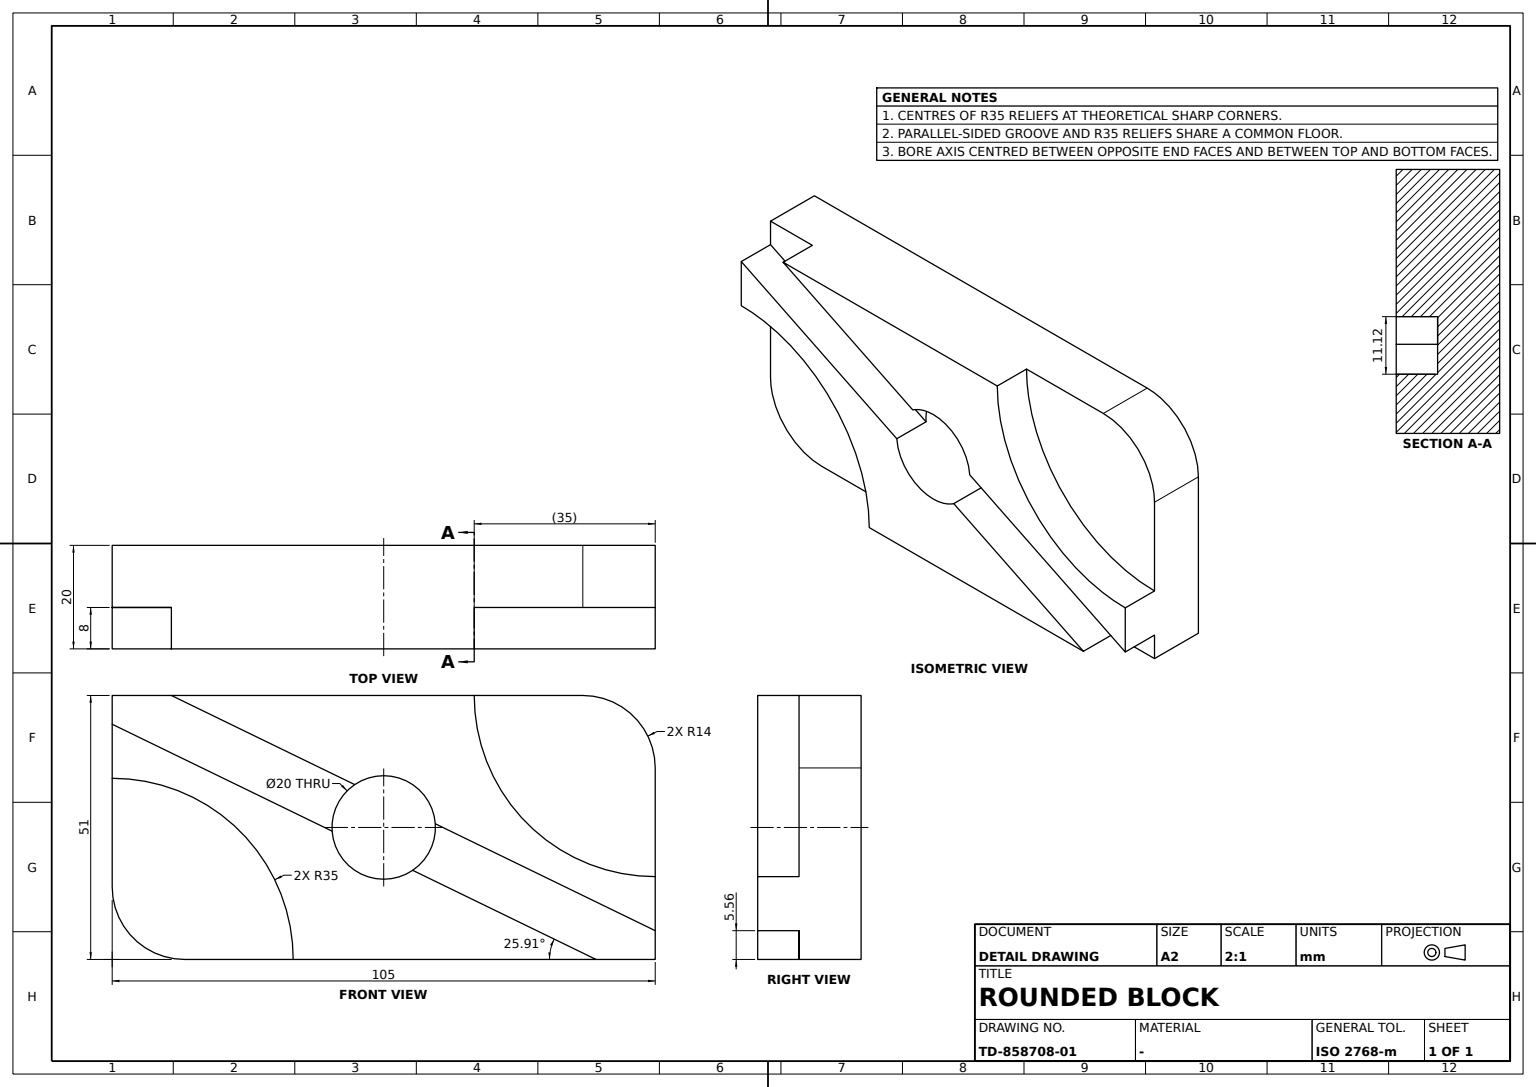
ISO-10303-21;
HEADER;
FILE_DESCRIPTION((''),'2;1');
FILE_NAME('','',(''),(''),'','','');
FILE_SCHEMA(('AUTOMOTIVE_DESIGN'));
ENDSEC;
DATA;
#1=APPLICATION_CONTEXT('');
#2=PRODUCT_CONTEXT('',#1,'mechanical');
#3=PRODUCT('','','',(#2));
#4=PRODUCT_DEFINITION_FORMATION('','',#3);
#5=PRODUCT_DEFINITION_CONTEXT('',#1,'design');
#6=PRODUCT_DEFINITION('','',#4,#5);
#7=PRODUCT_DEFINITION_SHAPE('','',#6);
#8=(LENGTH_UNIT()NAMED_UNIT(*)SI_UNIT(.MILLI.,.METRE.));
#9=(NAMED_UNIT(*)PLANE_ANGLE_UNIT()SI_UNIT($,.RADIAN.));
#10=(NAMED_UNIT(*)SI_UNIT($,.STERADIAN.)SOLID_ANGLE_UNIT());
#11=UNCERTAINTY_MEASURE_WITH_UNIT(LENGTH_MEASURE(0.005),#8,'distance_accuracy_value','');
#12=(GEOMETRIC_REPRESENTATION_CONTEXT(3)GLOBAL_UNCERTAINTY_ASSIGNED_CONTEXT((#11))GLOBAL_UNIT_ASSIGNED_CONTEXT((#8,#9,#10))REPRESENTATION_CONTEXT('',''));
#13=CARTESIAN_POINT('',(-38.5,-12.,-25.5));
#14=VERTEX_POINT('',#13);
#15=CARTESIAN_POINT('',(-52.5,-12.,-11.5));
#16=VERTEX_POINT('',#15);
#17=CARTESIAN_POINT('',(-38.5,-12.,-11.5));
#18=DIRECTION('',(0.,1.,0.));
#19=DIRECTION('',(0.,0.,-1.));
#20=AXIS2_PLACEMENT_3D('',#17,#18,#19);
#21=CIRCLE('',#20,14.);
#22=EDGE_CURVE('',#14,#16,#21,.T.);
#23=ORIENTED_EDGE('',*,*,#22,.T.);
#24=CARTESIAN_POINT('',(-52.5,0.,-11.5));
#25=VERTEX_POINT('',#24);
#26=DIRECTION('',(0.,-1.,0.));
#27=VECTOR('',#26,1000.);
#28=LINE('',#24,#27);
#29=EDGE_CURVE('',#25,#16,#28,.T.);
#30=ORIENTED_EDGE('',*,*,#29,.F.);
#31=CARTESIAN_POINT('',(-38.5,0.,-25.5));
#32=VERTEX_POINT('',#31);
#33=CARTESIAN_POINT('',(-38.5,0.,-11.5));
#34=DIRECTION('',(1.,0.,0.));
#35=AXIS2_PLACEMENT_3D('',#33,#26,#34);
#36=CIRCLE('',#35,14.);
#37=EDGE_CURVE('',#25,#32,#36,.T.);
#38=ORIENTED_EDGE('',*,*,#37,.T.);
#39=LINE('',#31,#27);
#40=EDGE_CURVE('',#32,#14,#39,.T.);
#41=ORIENTED_EDGE('',*,*,#40,.T.);
#42=EDGE_LOOP('',(#23,#30,#38,#41));
#43=FACE_BOUND('',#42,.T.);
#44=AXIS2_PLACEMENT_3D('',#33,#26,#19);
#45=CYLINDRICAL_SURFACE('',#44,14.);
#46=ADVANCED_FACE('',(#43),#45,.T.);
#47=CARTESIAN_POINT('',(-9.974489,-12.,-0.713841));
#48=VERTEX_POINT('',#47);
#49=CARTESIAN_POINT('',(-5.605449,-12.,8.28124));
#50=VERTEX_POINT('',#49);
#51=CARTESIAN_POINT('',(0.,-12.,0.));
#52=AXIS2_PLACEMENT_3D('',#51,#18,#19);
#53=CIRCLE('',#52,10.);
#54=EDGE_CURVE('',#48,#50,#53,.T.);
#55=ORIENTED_EDGE('',*,*,#54,.T.);
#56=CARTESIAN_POINT('',(-41.055837,-12.,25.5));
#57=VERTEX_POINT('',#56);
#58=DIRECTION('',(0.899508159,0.,-0.436903963));
#59=VECTOR('',#58,1000.);
#60=LINE('',#49,#59);
#61=EDGE_CURVE('',#57,#50,#60,.T.);
#62=ORIENTED_EDGE('',*,*,#61,.F.);
#63=CARTESIAN_POINT('',(-52.5,-12.,25.5));
#64=VERTEX_POINT('',#63);
#65=DIRECTION('',(-1.,0.,0.));
#66=VECTOR('',#65,1000.);
#67=LINE('',#56,#66);
#68=EDGE_CURVE('',#57,#64,#67,.T.);
#69=ORIENTED_EDGE('',*,*,#68,.T.);
#70=CARTESIAN_POINT('',(-52.5,-12.,19.941407));
#71=VERTEX_POINT('',#70);
#72=VECTOR('',#19,1000.);
#73=LINE('',#63,#72);
#74=EDGE_CURVE('',#64,#71,#73,.T.);
#75=ORIENTED_EDGE('',*,*,#74,.T.);
#76=DIRECTION('',(-0.899508159,0.,0.436903963));
#77=VECTOR('',#76,1000.);
#78=LINE('',#70,#77);
#79=EDGE_CURVE('',#48,#71,#78,.T.);
#80=ORIENTED_EDGE('',*,*,#79,.F.);
#81=EDGE_LOOP('',(#55,#62,#69,#75,#80));
#82=FACE_BOUND('',#81,.T.);
#83=AXIS2_PLACEMENT_3D('',#51,#26,#19);
#84=PLANE('',#83);
#85=ADVANCED_FACE('',(#82),#84,.T.);
#86=CARTESIAN_POINT('',(-52.5,-12.,9.5));
#87=VERTEX_POINT('',#86);
#88=CARTESIAN_POINT('',(-17.5,-12.,-25.5));
#89=VERTEX_POINT('',#88);
#90=CARTESIAN_POINT('',(-52.5,-12.,-25.5));
#91=AXIS2_PLACEMENT_3D('',#90,#18,#34);
#92=CIRCLE('',#91,35.);
#93=EDGE_CURVE('',#87,#89,#92,.T.);
#94=ORIENTED_EDGE('',*,*,#93,.F.);
#95=LINE('',#86,#72);
#96=EDGE_CURVE('',#87,#16,#95,.T.);
#97=ORIENTED_EDGE('',*,*,#96,.T.);
#98=ORIENTED_EDGE('',*,*,#22,.F.);
#99=VECTOR('',#34,1000.);
#100=LINE('',#90,#99);
#101=EDGE_CURVE('',#14,#89,#100,.T.);
#102=ORIENTED_EDGE('',*,*,#101,.T.);
#103=EDGE_LOOP('',(#94,#97,#98,#102));
#104=FACE_BOUND('',#103,.T.);
#105=AXIS2_PLACEMENT_3D('',#90,#26,#19);
#106=PLANE('',#105);
#107=ADVANCED_FACE('',(#104),#106,.T.);
#108=CARTESIAN_POINT('',(17.5,-20.,25.5));
#109=VERTEX_POINT('',#108);
#110=CARTESIAN_POINT('',(52.5,-20.,-9.5));
#111=VERTEX_POINT('',#110);
#112=CARTESIAN_POINT('',(52.5,-20.,25.5));
#113=AXIS2_PLACEMENT_3D('',#112,#26,#34);
#114=CIRCLE('',#113,35.);
#115=EDGE_CURVE('',#109,#111,#114,.T.);
#116=ORIENTED_EDGE('',*,*,#115,.F.);
#117=CARTESIAN_POINT('',(-41.055837,-20.,25.5));
#118=VERTEX_POINT('',#117);
#119=CARTESIAN_POINT('',(38.5,-20.,25.5));
#120=LINE('',#119,#66);
#121=EDGE_CURVE('',#109,#118,#120,.T.);
#122=ORIENTED_EDGE('',*,*,#121,.T.);
#123=CARTESIAN_POINT('',(-5.605449,-20.,8.28124));
#124=VERTEX_POINT('',#123);
#125=LINE('',#123,#77);
#126=EDGE_CURVE('',#124,#118,#125,.T.);
#127=ORIENTED_EDGE('',*,*,#126,.F.);
#128=CARTESIAN_POINT('',(0.,-20.,10.));
#129=VERTEX_POINT('',#128);
#130=CARTESIAN_POINT('',(0.,-20.,0.));
#131=AXIS2_PLACEMENT_3D('',#130,#26,#34);
#132=CIRCLE('',#131,10.);
#133=EDGE_CURVE('',#129,#124,#132,.T.);
#134=ORIENTED_EDGE('',*,*,#133,.F.);
#135=CARTESIAN_POINT('',(9.974489,-20.,0.713841));
#136=VERTEX_POINT('',#135);
#137=EDGE_CURVE('',#136,#129,#132,.T.);
#138=ORIENTED_EDGE('',*,*,#137,.F.);
#139=CARTESIAN_POINT('',(52.5,-20.,-19.941407));
#140=VERTEX_POINT('',#139);
#141=LINE('',#139,#77);
#142=EDGE_CURVE('',#140,#136,#141,.T.);
#143=ORIENTED_EDGE('',*,*,#142,.F.);
#144=CARTESIAN_POINT('',(52.5,-20.,-25.5));
#145=DIRECTION('',(0.,0.,1.));
#146=VECTOR('',#145,1000.);
#147=LINE('',#144,#146);
#148=EDGE_CURVE('',#140,#111,#147,.T.);
#149=ORIENTED_EDGE('',*,*,#148,.T.);
#150=EDGE_LOOP('',(#116,#122,#127,#134,#138,#143,#149));
#151=FACE_BOUND('',#150,.T.);
#152=CARTESIAN_POINT('',(-38.5,-20.,-11.5));
#153=AXIS2_PLACEMENT_3D('',#152,#26,#19);
#154=PLANE('',#153);
#155=ADVANCED_FACE('',(#151),#154,.T.);
#156=CARTESIAN_POINT('',(0.,0.,-10.));
#157=VERTEX_POINT('',#156);
#158=CARTESIAN_POINT('',(0.,-20.,-10.));
#159=VERTEX_POINT('',#158);
#160=LINE('',#156,#27);
#161=EDGE_CURVE('',#157,#159,#160,.T.);
#162=ORIENTED_EDGE('',*,*,#161,.T.);
#163=CARTESIAN_POINT('',(5.605449,-20.,-8.28124));
#164=VERTEX_POINT('',#163);
#165=EDGE_CURVE('',#159,#164,#132,.T.);
#166=ORIENTED_EDGE('',*,*,#165,.T.);
#167=CARTESIAN_POINT('',(5.605449,-12.,-8.28124));
#168=VERTEX_POINT('',#167);
#169=LINE('',#167,#27);
#170=EDGE_CURVE('',#168,#164,#169,.T.);
#171=ORIENTED_EDGE('',*,*,#170,.F.);
#172=CARTESIAN_POINT('',(9.974489,-12.,0.713841));
#173=VERTEX_POINT('',#172);
#174=EDGE_CURVE('',#173,#168,#53,.T.);
#175=ORIENTED_EDGE('',*,*,#174,.F.);
#176=LINE('',#172,#27);
#177=EDGE_CURVE('',#173,#136,#176,.T.);
#178=ORIENTED_EDGE('',*,*,#177,.T.);
#179=ORIENTED_EDGE('',*,*,#137,.T.);
#180=CARTESIAN_POINT('',(0.,0.,10.));
#181=VERTEX_POINT('',#180);
#182=LINE('',#180,#27);
#183=EDGE_CURVE('',#129,#181,#182,.F.);
#184=ORIENTED_EDGE('',*,*,#183,.T.);
#185=CARTESIAN_POINT('',(0.,0.,0.));
#186=AXIS2_PLACEMENT_3D('',#185,#26,#34);
#187=CIRCLE('',#186,10.);
#188=EDGE_CURVE('',#157,#181,#187,.T.);
#189=ORIENTED_EDGE('',*,*,#188,.F.);
#190=EDGE_LOOP('',(#162,#166,#171,#175,#178,#179,#184,#189));
#191=FACE_BOUND('',#190,.T.);
#192=AXIS2_PLACEMENT_3D('',#185,#26,#19);
#193=CYLINDRICAL_SURFACE('',#192,10.);
#194=ADVANCED_FACE('',(#191),#193,.F.);
#195=CARTESIAN_POINT('',(-9.974489,-20.,-0.713841));
#196=VERTEX_POINT('',#195);
#197=EDGE_CURVE('',#196,#159,#132,.T.);
#198=ORIENTED_EDGE('',*,*,#197,.T.);
#199=ORIENTED_EDGE('',*,*,#161,.F.);
#200=EDGE_CURVE('',#181,#157,#187,.T.);
#201=ORIENTED_EDGE('',*,*,#200,.F.);
#202=ORIENTED_EDGE('',*,*,#183,.F.);
#203=ORIENTED_EDGE('',*,*,#133,.T.);
#204=LINE('',#49,#27);
#205=EDGE_CURVE('',#50,#124,#204,.T.);
#206=ORIENTED_EDGE('',*,*,#205,.F.);
#207=ORIENTED_EDGE('',*,*,#54,.F.);
#208=LINE('',#47,#27);
#209=EDGE_CURVE('',#48,#196,#208,.T.);
#210=ORIENTED_EDGE('',*,*,#209,.T.);
#211=EDGE_LOOP('',(#198,#199,#201,#202,#203,#206,#207,#210));
#212=FACE_BOUND('',#211,.T.);
#213=ADVANCED_FACE('',(#212),#193,.F.);
#214=CARTESIAN_POINT('',(41.055837,-12.,-25.5));
#215=VERTEX_POINT('',#214);
#216=CARTESIAN_POINT('',(52.5,-12.,-25.5));
#217=VERTEX_POINT('',#216);
#218=LINE('',#214,#99);
#219=EDGE_CURVE('',#215,#217,#218,.T.);
#220=ORIENTED_EDGE('',*,*,#219,.T.);
#221=CARTESIAN_POINT('',(52.5,-12.,-19.941407));
#222=VERTEX_POINT('',#221);
#223=LINE('',#216,#146);
#224=EDGE_CURVE('',#217,#222,#223,.T.);
#225=ORIENTED_EDGE('',*,*,#224,.T.);
#226=LINE('',#221,#59);
#227=EDGE_CURVE('',#173,#222,#226,.T.);
#228=ORIENTED_EDGE('',*,*,#227,.F.);
#229=ORIENTED_EDGE('',*,*,#174,.T.);
#230=LINE('',#167,#77);
#231=EDGE_CURVE('',#215,#168,#230,.T.);
#232=ORIENTED_EDGE('',*,*,#231,.F.);
#233=EDGE_LOOP('',(#220,#225,#228,#229,#232));
#234=FACE_BOUND('',#233,.T.);
#235=ADVANCED_FACE('',(#234),#84,.T.);
#236=ORIENTED_EDGE('',*,*,#93,.T.);
#237=CARTESIAN_POINT('',(-17.5,-20.,-25.5));
#238=VERTEX_POINT('',#237);
#239=LINE('',#88,#27);
#240=EDGE_CURVE('',#89,#238,#239,.T.);
#241=ORIENTED_EDGE('',*,*,#240,.T.);
#242=CARTESIAN_POINT('',(-52.5,-20.,9.5));
#243=VERTEX_POINT('',#242);
#244=CARTESIAN_POINT('',(-52.5,-20.,-25.5));
#245=AXIS2_PLACEMENT_3D('',#244,#26,#34);
#246=CIRCLE('',#245,35.);
#247=EDGE_CURVE('',#238,#243,#246,.T.);
#248=ORIENTED_EDGE('',*,*,#247,.T.);
#249=LINE('',#86,#27);
#250=EDGE_CURVE('',#87,#243,#249,.T.);
#251=ORIENTED_EDGE('',*,*,#250,.F.);
#252=EDGE_LOOP('',(#236,#241,#248,#251));
#253=FACE_BOUND('',#252,.T.);
#254=CYLINDRICAL_SURFACE('',#105,35.);
#255=ADVANCED_FACE('',(#253),#254,.F.);
#256=CARTESIAN_POINT('',(52.5,-12.,-9.5));
#257=VERTEX_POINT('',#256);
#258=CARTESIAN_POINT('',(52.5,-12.,11.5));
#259=VERTEX_POINT('',#258);
#260=LINE('',#256,#146);
#261=EDGE_CURVE('',#257,#259,#260,.T.);
#262=ORIENTED_EDGE('',*,*,#261,.T.);
#263=CARTESIAN_POINT('',(38.5,-12.,25.5));
#264=VERTEX_POINT('',#263);
#265=CARTESIAN_POINT('',(38.5,-12.,11.5));
#266=AXIS2_PLACEMENT_3D('',#265,#18,#19);
#267=CIRCLE('',#266,14.);
#268=EDGE_CURVE('',#264,#259,#267,.T.);
#269=ORIENTED_EDGE('',*,*,#268,.F.);
#270=CARTESIAN_POINT('',(17.5,-12.,25.5));
#271=VERTEX_POINT('',#270);
#272=CARTESIAN_POINT('',(52.5,-12.,25.5));
#273=LINE('',#272,#66);
#274=EDGE_CURVE('',#264,#271,#273,.T.);
#275=ORIENTED_EDGE('',*,*,#274,.T.);
#276=AXIS2_PLACEMENT_3D('',#272,#18,#34);
#277=CIRCLE('',#276,35.);
#278=EDGE_CURVE('',#257,#271,#277,.T.);
#279=ORIENTED_EDGE('',*,*,#278,.F.);
#280=EDGE_LOOP('',(#262,#269,#275,#279));
#281=FACE_BOUND('',#280,.T.);
#282=AXIS2_PLACEMENT_3D('',#272,#26,#19);
#283=PLANE('',#282);
#284=ADVANCED_FACE('',(#281),#283,.T.);
#285=CARTESIAN_POINT('',(41.055837,-20.,-25.5));
#286=VERTEX_POINT('',#285);
#287=LINE('',#214,#27);
#288=EDGE_CURVE('',#215,#286,#287,.T.);
#289=ORIENTED_EDGE('',*,*,#288,.T.);
#290=CARTESIAN_POINT('',(-38.5,-20.,-25.5));
#291=LINE('',#290,#99);
#292=EDGE_CURVE('',#238,#286,#291,.T.);
#293=ORIENTED_EDGE('',*,*,#292,.F.);
#294=ORIENTED_EDGE('',*,*,#240,.F.);
#295=ORIENTED_EDGE('',*,*,#101,.F.);
#296=ORIENTED_EDGE('',*,*,#40,.F.);
#297=CARTESIAN_POINT('',(52.5,0.,-25.5));
#298=VERTEX_POINT('',#297);
#299=LINE('',#31,#99);
#300=EDGE_CURVE('',#32,#298,#299,.T.);
#301=ORIENTED_EDGE('',*,*,#300,.T.);
#302=LINE('',#297,#27);
#303=EDGE_CURVE('',#298,#217,#302,.T.);
#304=ORIENTED_EDGE('',*,*,#303,.T.);
#305=ORIENTED_EDGE('',*,*,#219,.F.);
#306=EDGE_LOOP('',(#289,#293,#294,#295,#296,#301,#304,#305));
#307=FACE_BOUND('',#306,.T.);
#308=AXIS2_PLACEMENT_3D('',#31,#19,#65);
#309=PLANE('',#308);
#310=ADVANCED_FACE('',(#307),#309,.T.);
#311=CARTESIAN_POINT('',(38.5,0.,25.5));
#312=VERTEX_POINT('',#311);
#313=LINE('',#311,#27);
#314=EDGE_CURVE('',#312,#264,#313,.T.);
#315=ORIENTED_EDGE('',*,*,#314,.T.);
#316=ORIENTED_EDGE('',*,*,#268,.T.);
#317=CARTESIAN_POINT('',(52.5,0.,11.5));
#318=VERTEX_POINT('',#317);
#319=LINE('',#317,#27);
#320=EDGE_CURVE('',#318,#259,#319,.T.);
#321=ORIENTED_EDGE('',*,*,#320,.F.);
#322=CARTESIAN_POINT('',(38.5,0.,11.5));
#323=AXIS2_PLACEMENT_3D('',#322,#26,#34);
#324=CIRCLE('',#323,14.);
#325=EDGE_CURVE('',#318,#312,#324,.T.);
#326=ORIENTED_EDGE('',*,*,#325,.T.);
#327=EDGE_LOOP('',(#315,#316,#321,#326));
#328=FACE_BOUND('',#327,.T.);
#329=AXIS2_PLACEMENT_3D('',#322,#26,#19);
#330=CYLINDRICAL_SURFACE('',#329,14.);
#331=ADVANCED_FACE('',(#328),#330,.T.);
#332=ORIENTED_EDGE('',*,*,#165,.F.);
#333=ORIENTED_EDGE('',*,*,#197,.F.);
#334=CARTESIAN_POINT('',(-52.5,-20.,19.941407));
#335=VERTEX_POINT('',#334);
#336=CARTESIAN_POINT('',(-45.424877,-20.,16.504918));
#337=LINE('',#336,#59);
#338=EDGE_CURVE('',#335,#196,#337,.T.);
#339=ORIENTED_EDGE('',*,*,#338,.F.);
#340=CARTESIAN_POINT('',(-52.5,-20.,25.5));
#341=LINE('',#340,#72);
#342=EDGE_CURVE('',#335,#243,#341,.T.);
#343=ORIENTED_EDGE('',*,*,#342,.T.);
#344=ORIENTED_EDGE('',*,*,#247,.F.);
#345=ORIENTED_EDGE('',*,*,#292,.T.);
#346=LINE('',#163,#59);
#347=EDGE_CURVE('',#164,#286,#346,.T.);
#348=ORIENTED_EDGE('',*,*,#347,.F.);
#349=EDGE_LOOP('',(#332,#333,#339,#343,#344,#345,#348));
#350=FACE_BOUND('',#349,.T.);
#351=ADVANCED_FACE('',(#350),#154,.T.);
#352=LINE('',#70,#27);
#353=EDGE_CURVE('',#71,#335,#352,.T.);
#354=ORIENTED_EDGE('',*,*,#353,.F.);
#355=ORIENTED_EDGE('',*,*,#74,.F.);
#356=CARTESIAN_POINT('',(-52.5,0.,25.5));
#357=VERTEX_POINT('',#356);
#358=LINE('',#356,#27);
#359=EDGE_CURVE('',#357,#64,#358,.T.);
#360=ORIENTED_EDGE('',*,*,#359,.F.);
#361=LINE('',#356,#72);
#362=EDGE_CURVE('',#357,#25,#361,.T.);
#363=ORIENTED_EDGE('',*,*,#362,.T.);
#364=ORIENTED_EDGE('',*,*,#29,.T.);
#365=ORIENTED_EDGE('',*,*,#96,.F.);
#366=ORIENTED_EDGE('',*,*,#250,.T.);
#367=ORIENTED_EDGE('',*,*,#342,.F.);
#368=EDGE_LOOP('',(#354,#355,#360,#363,#364,#365,#366,#367));
#369=FACE_BOUND('',#368,.T.);
#370=AXIS2_PLACEMENT_3D('',#356,#65,#145);
#371=PLANE('',#370);
#372=ADVANCED_FACE('',(#369),#371,.T.);
#373=ORIENTED_EDGE('',*,*,#338,.T.);
#374=ORIENTED_EDGE('',*,*,#209,.F.);
#375=ORIENTED_EDGE('',*,*,#79,.T.);
#376=ORIENTED_EDGE('',*,*,#353,.T.);
#377=EDGE_LOOP('',(#373,#374,#375,#376));
#378=FACE_BOUND('',#377,.T.);
#379=CARTESIAN_POINT('',(-45.424877,-12.,16.504918));
#380=DIRECTION('',(-0.436903963,0.,-0.899508159));
#381=AXIS2_PLACEMENT_3D('',#379,#380,#76);
#382=PLANE('',#381);
#383=ADVANCED_FACE('',(#378),#382,.F.);
#384=LINE('',#270,#27);
#385=EDGE_CURVE('',#271,#109,#384,.T.);
#386=ORIENTED_EDGE('',*,*,#385,.T.);
#387=ORIENTED_EDGE('',*,*,#115,.T.);
#388=LINE('',#256,#27);
#389=EDGE_CURVE('',#257,#111,#388,.T.);
#390=ORIENTED_EDGE('',*,*,#389,.F.);
#391=ORIENTED_EDGE('',*,*,#278,.T.);
#392=EDGE_LOOP('',(#386,#387,#390,#391));
#393=FACE_BOUND('',#392,.T.);
#394=CYLINDRICAL_SURFACE('',#282,35.);
#395=ADVANCED_FACE('',(#393),#394,.F.);
#396=ORIENTED_EDGE('',*,*,#227,.T.);
#397=LINE('',#221,#27);
#398=EDGE_CURVE('',#222,#140,#397,.T.);
#399=ORIENTED_EDGE('',*,*,#398,.T.);
#400=ORIENTED_EDGE('',*,*,#142,.T.);
#401=ORIENTED_EDGE('',*,*,#177,.F.);
#402=EDGE_LOOP('',(#396,#399,#400,#401));
#403=FACE_BOUND('',#402,.T.);
#404=DIRECTION('',(0.436903963,0.,0.899508159));
#405=AXIS2_PLACEMENT_3D('',#221,#404,#58);
#406=PLANE('',#405);
#407=ADVANCED_FACE('',(#403),#406,.F.);
#408=ORIENTED_EDGE('',*,*,#148,.F.);
#409=ORIENTED_EDGE('',*,*,#398,.F.);
#410=ORIENTED_EDGE('',*,*,#224,.F.);
#411=ORIENTED_EDGE('',*,*,#303,.F.);
#412=LINE('',#297,#146);
#413=EDGE_CURVE('',#298,#318,#412,.T.);
#414=ORIENTED_EDGE('',*,*,#413,.T.);
#415=ORIENTED_EDGE('',*,*,#320,.T.);
#416=ORIENTED_EDGE('',*,*,#261,.F.);
#417=ORIENTED_EDGE('',*,*,#389,.T.);
#418=EDGE_LOOP('',(#408,#409,#410,#411,#414,#415,#416,#417));
#419=FACE_BOUND('',#418,.T.);
#420=AXIS2_PLACEMENT_3D('',#297,#34,#19);
#421=PLANE('',#420);
#422=ADVANCED_FACE('',(#419),#421,.T.);
#423=LINE('',#56,#27);
#424=EDGE_CURVE('',#57,#118,#423,.T.);
#425=ORIENTED_EDGE('',*,*,#424,.F.);
#426=ORIENTED_EDGE('',*,*,#61,.T.);
#427=ORIENTED_EDGE('',*,*,#205,.T.);
#428=ORIENTED_EDGE('',*,*,#126,.T.);
#429=EDGE_LOOP('',(#425,#426,#427,#428));
#430=FACE_BOUND('',#429,.T.);
#431=AXIS2_PLACEMENT_3D('',#49,#404,#58);
#432=PLANE('',#431);
#433=ADVANCED_FACE('',(#430),#432,.F.);
#434=ORIENTED_EDGE('',*,*,#170,.T.);
#435=ORIENTED_EDGE('',*,*,#347,.T.);
#436=ORIENTED_EDGE('',*,*,#288,.F.);
#437=ORIENTED_EDGE('',*,*,#231,.T.);
#438=EDGE_LOOP('',(#434,#435,#436,#437));
#439=FACE_BOUND('',#438,.T.);
#440=AXIS2_PLACEMENT_3D('',#167,#380,#76);
#441=PLANE('',#440);
#442=ADVANCED_FACE('',(#439),#441,.F.);
#443=ORIENTED_EDGE('',*,*,#300,.F.);
#444=ORIENTED_EDGE('',*,*,#37,.F.);
#445=ORIENTED_EDGE('',*,*,#362,.F.);
#446=LINE('',#311,#66);
#447=EDGE_CURVE('',#312,#357,#446,.T.);
#448=ORIENTED_EDGE('',*,*,#447,.F.);
#449=ORIENTED_EDGE('',*,*,#325,.F.);
#450=ORIENTED_EDGE('',*,*,#413,.F.);
#451=EDGE_LOOP('',(#443,#444,#445,#448,#449,#450));
#452=FACE_BOUND('',#451,.T.);
#453=ORIENTED_EDGE('',*,*,#200,.T.);
#454=ORIENTED_EDGE('',*,*,#188,.T.);
#455=EDGE_LOOP('',(#453,#454));
#456=FACE_BOUND('',#455,.T.);
#457=PLANE('',#44);
#458=ADVANCED_FACE('',(#452,#456),#457,.F.);
#459=ORIENTED_EDGE('',*,*,#385,.F.);
#460=ORIENTED_EDGE('',*,*,#274,.F.);
#461=ORIENTED_EDGE('',*,*,#314,.F.);
#462=ORIENTED_EDGE('',*,*,#447,.T.);
#463=ORIENTED_EDGE('',*,*,#359,.T.);
#464=ORIENTED_EDGE('',*,*,#68,.F.);
#465=ORIENTED_EDGE('',*,*,#424,.T.);
#466=ORIENTED_EDGE('',*,*,#121,.F.);
#467=EDGE_LOOP('',(#459,#460,#461,#462,#463,#464,#465,#466));
#468=FACE_BOUND('',#467,.T.);
#469=AXIS2_PLACEMENT_3D('',#311,#145,#34);
#470=PLANE('',#469);
#471=ADVANCED_FACE('',(#468),#470,.T.);
#472=CLOSED_SHELL('',(#46,#85,#107,#155,#194,#213,#235,#255,#284,#310,#331,#351,#372,#383,#395,#407,#422,#433,#442,#458,#471));
#473=MANIFOLD_SOLID_BREP('',#472);
#474=ADVANCED_BREP_SHAPE_REPRESENTATION('',(#473),#12);
#475=SHAPE_DEFINITION_REPRESENTATION(#7,#474);
ENDSEC;
END-ISO-10303-21;
